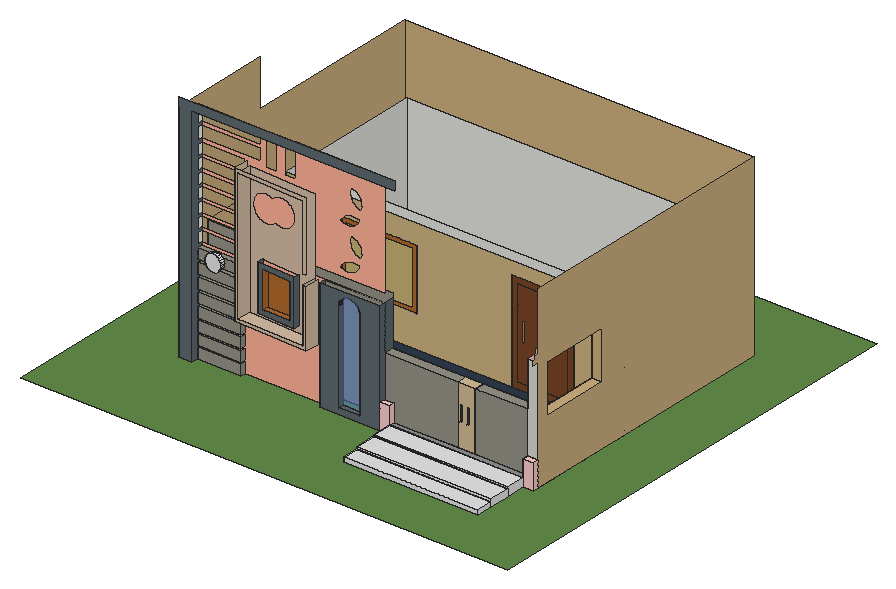
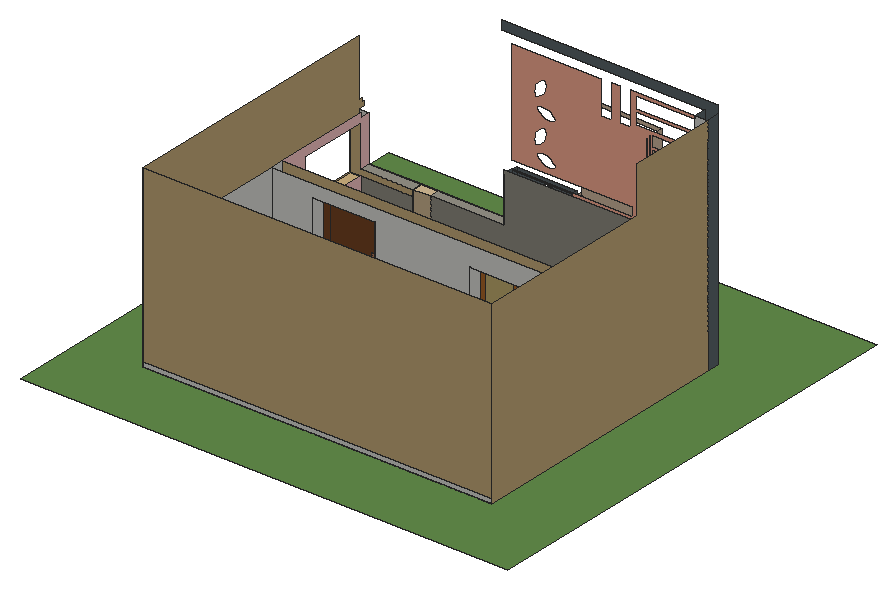
# SketchUp Ruby script. Lengths in inches.
U = 1.inch
M = Sketchup.active_model
def pt(a) = Geom::Point3d.new(a.map { |v| v * U })
def face(e, loops, mat)
  f = e.add_face(loops[0].map { |a| pt(a) })
  loops[1..].each { |l| e.add_face(l.map { |a| pt(a) }).erase! }
  f.material = f.back_material = mat if mat
  f
end
# faces: each face lists its corners as indices into pts; further lists are holes
def faces(e, pts, list, mat = nil) = list.each { |f| face(e, (f[0].is_a?(Array) ? f : [f]).map { |l| l.map { |i| pts[i] } }, mat) }
# xy, xz, yz: faces in a plane at the given z, y or x. An outline is a flat list of corners, or four numbers for a rectangle; further outlines are holes
def ring(l) = l.size == 4 ? [[l[0], l[1]], [l[2], l[1]], [l[2], l[3]], [l[0], l[3]]] : l.each_slice(2).to_a
def flat(e, list, mat, &to3) = list.each { |f| face(e, (f[0].is_a?(Array) ? f : [f]).map { |l| ring(l).map { |u, v| to3.(u, v) } }, mat) }
def xy(e, z, list, mat = nil) = flat(e, list, mat) { |x, y| [x, y, z] }
def xz(e, y, list, mat = nil) = flat(e, list, mat) { |x, z| [x, y, z] }
def yz(e, x, list, mat = nil) = flat(e, list, mat) { |y, z| [x, y, z] }
def lines(e, pts, list) = list.each { |a, b| e.add_line(pt(pts[a]), pt(pts[b])) }
# prism: a flat outline (further loops are holes) pulled along v
def prism(e, loops, v, mat = nil)
  f = face(e, loops, mat); d = Geom::Vector3d.new(v.map { |x| x * U })
  f.pushpull(f.normal.samedirection?(d) ? d.length : -d.length)
end
def box(e, o, s, mat = nil) = prism(e, [[o, [o[0] + s[0], o[1], o[2]], [o[0] + s[0], o[1] + s[1], o[2]], [o[0], o[1] + s[1], o[2]]]], [0, 0, s[2]], mat)
def at(x, y, z, deg = 0) = Geom::Transformation.translation(pt([x, y, z])) * Geom::Transformation.rotation(ORIGIN, Z_AXIS, deg.degrees)
def axes(o, x, y, z) = Geom::Transformation.new([*x, 0, *y, 0, *z, 0, *pt(o).to_a, 1])
def part(name) = M.definitions.add(name)
# library, detail: a bought-in or finely detailed component or shape, given as its bounding box
def library(name, o, s) = part(name).tap { |d| box(d.entities, o, s) }
def detail(e, o, s) = box(e.add_group.entities, o, s)
def put(e, d, t, mat = nil) = e.add_instance(d, t).tap { |i| i.material = mat if mat }
def group(e, t, mat = nil) = e.add_group.tap { |g| g.transformation = t; g.material = mat if mat }.entities
root = M.entities
M.materials.add("[Blacktop Old 02]").color = [143, 145, 145]
M.materials.add("[Color A01]").color = [255, 204, 204]
M.materials.add("[Color B02]").color = [255, 178, 153]
M.materials.add("[Formica Beige]").color = [211, 187, 149]
M.materials.add("[Formica Graystone]").color = [149, 146, 135]
M.materials.add("[Formica Laminate Dark]").color = [50, 53, 60]
M.materials.add("[Formica Laminate Light]").color = [213, 189, 164]
M.materials.add("[Formica Speckled Grey]").color = [94, 105, 111]
M.materials.add("[Leather Blue]").color = [45, 57, 74]
M.materials.add("[Polished Concrete Old]").color = [229, 229, 229]
M.materials.add("[Stone Sandstone Ashlar Light]").color = [206, 178, 128]
M.materials.add("[Terrazzo Tile Light]").color = [219, 217, 210]
M.materials.add("[Translucent Glass Blue]").color = [100, 149, 237]
M.materials["[Translucent Glass Blue]"].alpha = 0.5
M.materials.add("[Vegetation Grass Artificial]").color = [98, 140, 74]
M.materials.add("[Window Covering 02]").color = [199, 178, 115]
M.materials.add("[Wood Bamboo]").color = [177, 105, 43]
M.materials.add("[Wood Floor Light]").color = [204, 176, 127]
M.materials.add("[Wood Veneer 01]").color = [120, 70, 37]
M.materials.add("[Wood Veneer 02]").color = [190, 128, 91]
xy(root,0,[[652.51,124.47,963.43,160.81],[652.51,160.81,963.43,210.65],[652.51,210.65,963.43,256.01],[176.71,240.39,205.21,269.01],[491.29,256.01,491.29,269.01,307.34,269.01,307.34,257.39,205.21,257.39,205.21,269.01,176.71,269.01,176.71,894.96,987.53,894.96,987.53,256.01]])
xy(root,0,[[[0,0,1133.3125,1068.5625],[652.51,124.47,963.43,256.01],[176.71,240.39,205.21,269.01]]],"[Vegetation Grass Artificial]")
xy(root,9,[[963.43,269.01,987.53,293.12],[200.82,520.41,724.72,550.03],[724.72,520.41,868.85,550.03],[868.85,520.41,963.43,550.03],[200.82,550.03,963.43,870.85]])
xy(root,9,[[200.82,293.12,963.43,520.41]],"[Leather Blue]")
xy(root,10.8125,[[652.51,124.47,963.43,160.81]],"[Polished Concrete Old]")
xy(root,13.61,[[533.89,256.01,583.26,269.01]],"[Formica Speckled Grey]")
xy(root,15.875,[[652.51,160.81,963.43,210.65]],"[Polished Concrete Old]")
xy(root,19.25,[[652.51,256.01,963.43,269.01]],"[Blacktop Old 02]")
xy(root,19.25,[[841.49,269.01,963.43,293.12]],"[Color A01]")
xy(root,19.25,[[652.51,210.65,963.43,256.01]],"[Polished Concrete Old]")
xy(root,24,[[205.21,257.39,307.34,269.01]],"[Formica Graystone]")
xy(root,27.52,[[205.21,257.39,307.34,269.01]],"[Formica Graystone]")
xy(root,51.52,[[205.21,257.39,307.34,269.01]],"[Formica Graystone]")
xy(root,56.52,[[205.21,257.39,307.34,269.01]],"[Formica Graystone]")
xy(root,59.0625,[[630.73,256.01,652.51,269.01],[963.43,256.01,987.53,269.01]],"[Color A01]")
xy(root,80.52,[[205.21,257.39,307.34,269.01]],"[Formica Graystone]")
xy(root,83.125,[[330.4375,520.41,503.625,550.03]])
xy(root,85.21,[[205.21,257.39,307.34,269.01]],"[Formica Graystone]")
xy(root,109.21,[[205.21,257.39,307.34,269.01]],"[Formica Graystone]")
xy(root,115.21,[[205.21,257.39,307.34,269.01]],"[Formica Graystone]")
xy(root,124.35,[[479.36,228.58,309.09,236.05,310.54,269.01,480.8,261.55]],"[Formica Laminate Light]")
xy(root,131.76,[[471.96,228.91,473.4,261.88,317.94,268.69,316.5,235.72]],"[Formica Laminate Light]")
xy(root,139.21,[[205.21,257.39,307.34,269.01]],"[Formica Graystone]")
xy(root,140.16,[[963.43,293.12,987.53,454.16]],"[Wood Floor Light]")
xy(root,145.83,[[205.21,257.39,307.34,269.01]],"[Formica Graystone]")
xy(root,146.87,[[436.06,250.0625,348.76,253.89,349.35,267.3125,436.64,263.49]],"[Formica Speckled Grey]")
xy(root,155.65,[[800.41,269.01,841.49,293.12]],"[Formica Beige]")
xy(root,155.65,[[630.73,269.01,800.41,293.12],[841.49,269.01,963.43,293.12]],"[Formica Graystone]")
xy(root,158.32,[[424.62,250.56,425.21,263.99,360.79,266.8125,360.2,253.39]],"[Wood Bamboo]")
xy(root,169.83,[[205.21,257.39,307.34,269.01]],"[Formica Graystone]")
xy(root,176.46,[[205.21,257.39,307.34,269.01]],"[Formica Graystone]")
xy(root,200.46,[[205.21,257.39,307.34,269.01]],"[Formica Graystone]")
xy(root,225.3125,[[330.4375,520.41,503.625,550.03]])
xy(root,231.08,[[205.21,257.39,307.34,269.01]],"[Formica Graystone]")
xz(root,124.47,[[652.51,0,963.43,10.8125]],"[Polished Concrete Old]")
xz(root,160.81,[[652.51,0,963.43,10.8125]])
xz(root,160.81,[[652.51,10.8125,963.43,15.875]],"[Polished Concrete Old]")
xz(root,210.65,[[652.51,0,963.43,15.875]])
xz(root,210.65,[[652.51,15.875,963.43,19.25]],"[Polished Concrete Old]")
xz(root,240.39,[[176.71,0,205.21,0,205.21,522.12,678.16,522.12,678.16,542.5625,176.71,542.5625]],"[Formica Speckled Grey]")
xz(root,246.45,[[249.96,200.625,254.76,201.25,259.24,203.11,263.08,206.05,263.87,207.08,266.02,209.89,267.875,214.37,268.51,219.17,267.875,223.97,266.02,228.4375,263.99,231.08,263.08,232.28,259.24,235.23,254.76,237.08,249.96,237.71,245.16,237.08,240.69,235.23,236.85,232.28,235.94,231.08,233.9,228.4375,232.05,223.97,231.42,219.17,232.05,214.37,233.9,209.89,236.0625,207.08,236.85,206.05,240.69,203.11,245.16,201.25]],"[Polished Concrete Old]")
xz(root,256.01,[[630.73,0,652.51,59.0625],[963.43,0,987.53,59.0625]],"[Color A01]")
xz(root,256.01,[[[491.29,0,630.73,259.36],[533.89,13.61,533.89,224.73,533.92,226.02,534.02,227.3125,534.19,228.59,534.43,229.86,534.73,231.12,535.1,232.36,535.53,233.58,536.02,234.77,536.58,235.9375,537.2,237.07,537.87,238.18,538.6,239.24,539.39,240.27,540.23,241.25,541.12,242.1875,542.06,243.08,543.04,243.92,544.07,244.7,545.13,245.4375,546.23,246.11,547.37,246.73,548.54,247.28,549.73,247.78,550.95,248.21,552.1875,248.58,553.44,248.88,554.72,249.11,556,249.28,557.29,249.38,558.58,249.42,559.87,249.38,561.16,249.28,562.4375,249.11,563.71,248.88,564.97,248.58,566.21,248.21,567.42,247.78,568.62,247.28,569.79,246.73,570.92,246.11,572.02,245.4375,573.09,244.7,574.11,243.92,575.1,243.08,576.03,242.1875,576.92,241.25,577.76,240.27,578.55,239.24,579.28,238.18,579.96,237.07,580.57,235.9375,581.13,234.77,581.625,233.58,582.06,232.36,582.42,231.12,582.73,229.86,582.96,228.59,583.13,227.3125,583.23,226.02,583.26,224.73,583.26,13.61]],[652.51,0,963.43,19.25]],"[Formica Speckled Grey]")
xz(root,257.39,[[235.94,231.08,236.85,232.28,240.69,235.23,245.16,237.08,249.96,237.71,254.76,237.08,259.24,235.23,263.08,232.28,263.99,231.08]])
xz(root,257.39,[[205.21,0,307.34,24],[205.21,27.52,307.34,51.52],[205.21,56.52,307.34,80.52],[205.21,85.21,307.34,109.21],[205.21,115.21,307.34,139.21],
  [205.21,145.83,307.34,169.83],[205.21,176.46,307.34,200.46],[205.21,207.08,236.0625,207.08,233.9,209.89,232.05,214.37,231.42,219.17,232.05,223.97,233.9,228.4375,235.94,231.08,205.21,231.08],[263.87,207.08,307.34,207.08,307.34,231.08,263.99,231.08,266.02,228.4375,267.875,223.97,268.51,219.17,267.875,214.37,266.02,209.89]],"[Formica Graystone]")
xz(root,269.01,[[176.71,0,205.21,522.12],[963.43,9,987.53,59.0625]])
xz(root,269.01,[[[307.34,0,491.29,0,491.29,259.36,630.73,259.36,630.73,261.0625,350.6,261.0625,350.6,280.3125,630.73,280.3125,630.73,522.12,424.625,522.12,424.625,445.43,399.125,445.43,399.125,522.12,380.1875,522.12,380.1875,445.43,354.6875,445.43,354.6875,522.12,205.21,522.12,205.21,515.1,342.46,515.1,342.46,488.66,205.21,488.66,205.21,481.6,342.46,481.6,342.46,455.16,205.21,455.16,205.21,445.46,307.34,445.46,307.34,421.46,205.21,421.46,205.21,414.83,307.34,414.83,307.34,390.83,205.21,390.83,205.21,384.21,307.34,384.21,307.34,360.21,205.21,360.21,205.21,353.58,307.34,353.58,307.34,329.58,205.21,329.58,205.21,322.96,307.34,322.96,307.34,298.96,205.21,298.96,205.21,292.33,307.34,292.33,307.34,268.33,205.21,268.33,205.21,261.71,307.34,261.71,307.34,237.71,205.21,237.71,205.21,231.08,307.34,231.08,307.34,207.08,205.21,207.08,205.21,200.46,307.34,200.46,307.34,176.46,205.21,176.46,205.21,169.83,307.34,169.83,307.34,145.83,205.21,145.83,205.21,139.21,307.34,139.21,307.34,115.21,205.21,115.21,205.21,109.21,307.34,109.21,307.34,85.21,205.21,85.21,205.21,80.52,307.34,80.52,307.34,56.52,205.21,56.52,205.21,51.52,307.34,51.52,307.34,27.52,205.21,27.52,205.21,24,307.34,24],[545.83,390.61,541.09,390.87,536.44,391.87,532.01,393.57,527.89,395.95,530.06,399.98,532.74,403.67,535.9,406.98,539.47,409.82,543.39,412.17,547.59,413.96,551.99,415.17,556.52,415.78,561.09,415.78,565.61,415.16,570.02,413.94,574.21,412.13,572.47,407.71,570.07,403.61,567.05,399.94,563.5,396.78,559.51,394.21,555.16,392.3,550.5625,391.09],[545.83,293.67,541.09,293.93,536.44,294.93,532.01,296.64,527.89,299.02,530.06,303.04,532.74,306.74,535.9,310.04,539.47,312.89,543.39,315.23,547.59,317.02,551.99,318.23,556.52,318.84,561.09,318.84,565.61,318.22,570.02,317,574.21,315.2,572.47,310.77,570.07,306.68,567.05,303,563.5,299.84,559.51,297.28,555.16,295.36,550.5625,294.15],[577.86,330.87,573.2,331.8,568.74,333.44,564.59,335.76,560.86,338.69,557.62,342.17,554.97,346.12,552.96,350.42,551.65,354.99,551.07,359.71,551.23,364.46,552.125,369.125,553.74,373.59,558.08,372.18,562.19,370.19,566,367.67,569.4375,364.66,572.4375,361.21,574.95,357.4,576.92,353.28,578.32,348.93,579.125,344.43,579.32,339.87,578.89,335.32],[577.86,431.06,573.2,431.99,568.74,433.63,564.59,435.95,560.86,438.88,557.62,442.36,554.97,446.3,552.96,450.61,551.65,455.18,551.07,459.89,551.23,464.64,552.125,469.3125,553.74,473.78,558.08,472.37,562.19,470.38,566,467.86,569.4375,464.85,572.4375,461.4,574.95,457.59,576.92,453.47,578.32,449.12,579.125,444.62,579.32,440.06,578.89,435.51]]],"[Color B02]")
xz(root,269.01,[[[800.41,19.25,841.49,155.65],[805.56,73.97,811.87,111.16],[821.68,73.97,827.99,111.16]]],"[Formica Beige]")
xz(root,269.01,[[652.51,19.25,800.41,19.25,800.41,155.65,630.73,155.65,630.73,59.0625,652.51,59.0625],[841.49,19.25,963.43,155.65]],"[Formica Graystone]")
xz(root,269.01,[[805.56,73.97,811.87,111.16],[821.68,73.97,827.99,111.16]],"[Formica Laminate Dark]")
xz(root,269.01,[[963.43,59.0625,987.53,261.0625]],"[Terrazzo Tile Light]")
xz(root,269.01,[[533.89,13.61,583.26,13.61,583.26,224.73,583.23,226.02,583.13,227.3125,582.96,228.59,582.73,229.86,582.42,231.12,582.06,232.36,581.625,233.58,581.13,234.77,580.57,235.9375,579.96,237.07,579.28,238.18,578.55,239.24,577.76,240.27,576.92,241.25,576.03,242.1875,575.1,243.08,574.11,243.92,573.09,244.7,572.02,245.4375,570.92,246.11,569.79,246.73,568.62,247.28,567.42,247.78,566.21,248.21,564.97,248.58,563.71,248.88,562.4375,249.11,561.16,249.28,559.87,249.38,558.58,249.42,557.29,249.38,556,249.28,554.72,249.11,553.44,248.88,552.1875,248.58,550.95,248.21,549.73,247.78,548.54,247.28,547.37,246.73,546.23,246.11,545.13,245.4375,544.07,244.7,543.04,243.92,542.06,243.08,541.12,242.1875,540.23,241.25,539.39,240.27,538.6,239.24,537.87,238.18,537.2,237.07,536.58,235.9375,536.02,234.77,535.53,233.58,535.1,232.36,534.73,231.12,534.43,229.86,534.19,228.59,534.02,227.3125,533.92,226.02,533.89,224.73]],"[Translucent Glass Blue]")
xz(root,293.12,[[963.43,9,987.53,140.16]])
xz(root,293.12,[[630.73,9,630.73,19.25,800.41,19.25,800.41,155.65,841.49,155.65,841.49,19.25,963.43,19.25,963.43,9]],"[Formica Beige]")
xz(root,293.12,[[200.82,9,200.82,271.3125,630.73,271.3125,630.73,155.65,800.41,155.65,800.41,19.25,630.73,19.25,630.73,9],[841.49,19.25,963.43,140.16]],"[Formica Graystone]")
xz(root,293.12,[[841.49,140.16,841.49,155.65,963.43,155.65,963.43,251.7,987.53,251.7,987.53,140.16]],"[Wood Floor Light]")
xz(root,454.16,[[963.43,140.16,987.53,251.7]],"[Wood Floor Light]")
xz(root,520.41,[[[200.82,9,724.72,9,724.72,242.2,868.85,242.2,868.85,9,963.43,9,963.43,271.3125,200.82,271.3125],[330.4375,83.125,503.625,225.3125]]],"[Stone Sandstone Ashlar Light]")
xz(root,520.41,[[340.5625,93.25,409.01,215.1875],[425.5,93.25,493.5,215.1875]],"[Window Covering 02]")
xz(root,520.41,[[[330.4375,83.125,503.625,225.3125],[340.5625,93.25,493.5,215.1875]],[409.01,93.25,425.5,215.1875]],"[Wood Bamboo]")
xz(root,520.41,[[[724.72,9,868.85,242.2],[739.6875,23.96,853.88,227.23]],[[739.6875,23.96,853.88,227.23],[747.59,107.64,755.03,154.64]]],"[Wood Veneer 01]")
xz(root,520.41,[[747.59,107.64,755.03,154.64]],"[Wood Veneer 02]")
xz(root,550.03,[[[200.82,9,200.82,271.3125,963.43,271.3125,963.43,9,868.85,9,868.85,242.2,724.72,242.2,724.72,9],[330.4375,83.125,503.625,225.3125]]])
xz(root,870.85,[[200.82,9,963.43,271.3125]])
xz(root,894.96,[[176.71,0,987.53,9]])
xz(root,894.96,[[176.71,9,987.53,414.1875]],"[Wood Floor Light]")
yz(root,176.71,[[240.39,0,269.01,522.12]],"[Formica Speckled Grey]")
yz(root,176.71,[[269.01,0,269.01,522.12,475.31,522.12,475.31,414.1875,894.96,414.1875,894.96,0]],"[Wood Floor Light]")
yz(root,200.82,[[520.41,9,550.03,271.3125],[550.03,9,870.85,271.3125]])
yz(root,200.82,[[293.12,9,520.41,271.3125]],"[Stone Sandstone Ashlar Light]")
yz(root,205.21,[[257.39,0,269.01,24],[257.39,27.52,269.01,51.52],[257.39,56.52,269.01,80.52],[257.39,85.21,269.01,109.21],[257.39,115.21,269.01,139.21],
  [257.39,145.83,269.01,169.83],[257.39,176.46,269.01,200.46],[257.39,207.08,269.01,231.08]])
yz(root,205.21,[[240.39,0,257.39,0,257.39,24,269.01,24,269.01,27.52,257.39,27.52,257.39,51.52,269.01,51.52,269.01,56.52,257.39,56.52,257.39,80.52,269.01,80.52,269.01,85.21,257.39,85.21,257.39,109.21,269.01,109.21,269.01,115.21,257.39,115.21,257.39,139.21,269.01,139.21,269.01,145.83,257.39,145.83,257.39,169.83,269.01,169.83,269.01,176.46,257.39,176.46,257.39,200.46,269.01,200.46,269.01,207.08,257.39,207.08,257.39,231.08,269.01,231.08,269.01,237.71,257.39,237.71,257.39,261.71,269.01,261.71,269.01,268.33,257.39,268.33,257.39,292.33,269.01,292.33,269.01,298.96,257.39,298.96,257.39,322.96,269.01,322.96,269.01,329.58,257.39,329.58,257.39,353.58,269.01,353.58,269.01,360.21,257.39,360.21,257.39,384.21,269.01,384.21,269.01,390.83,257.39,390.83,257.39,414.83,269.01,414.83,269.01,421.46,257.39,421.46,257.39,445.46,269.01,445.46,269.01,455.16,257.39,455.16,257.39,481.6,269.01,481.6,269.01,488.66,257.39,488.66,257.39,515.1,269.01,515.1,269.01,522.12,240.39,522.12]],"[Formica Speckled Grey]")
yz(root,307.34,[[257.39,145.83,269.01,169.83],[257.39,176.46,269.01,200.46],[257.39,207.08,269.01,231.08]])
yz(root,307.34,[[257.39,0,269.01,24],[257.39,27.52,269.01,51.52],[257.39,56.52,269.01,80.52],[257.39,85.21,269.01,109.21],[257.39,115.21,269.01,139.21]],"[Formica Graystone]")
yz(root,330.4375,[[520.41,83.125,550.03,225.3125]])
yz(root,491.29,[[256.01,0,269.01,259.36]],"[Formica Speckled Grey]")
yz(root,503.625,[[520.41,83.125,550.03,225.3125]])
yz(root,533.89,[[256.01,13.61,269.01,224.73]],"[Formica Speckled Grey]")
yz(root,583.26,[[256.01,13.61,269.01,224.73]],"[Formica Speckled Grey]")
yz(root,630.73,[[256.01,59.0625,269.01,259.36],[269.01,155.65,293.12,261.0625]],"[Formica Speckled Grey]")
yz(root,652.51,[[256.01,19.25,269.01,59.0625]],"[Color A01]")
yz(root,652.51,[[124.47,0,160.81,10.8125],[160.81,0,210.65,15.875],[210.65,0,256.01,19.25]],"[Polished Concrete Old]")
yz(root,724.72,[[520.41,9,550.03,242.2]])
yz(root,841.49,[[269.01,19.25,293.12,155.65]],"[Color A01]")
yz(root,868.85,[[520.41,9,550.03,242.2]])
yz(root,963.43,[[269.01,9,293.12,19.25],[520.41,9,550.03,271.3125],[550.03,9,870.85,271.3125]])
yz(root,963.43,[[293.12,9,293.12,140.16,454.16,140.16,454.16,251.7,293.12,251.7,293.12,155.65,269.01,155.65,269.01,261.0625,293.12,261.0625,293.12,271.3125,520.41,271.3125,520.41,9],[256.01,19.25,269.01,59.0625]],"[Color A01]")
yz(root,963.43,[[124.47,0,160.81,10.8125],[160.81,0,210.65,15.875],[210.65,0,256.01,19.25]],"[Polished Concrete Old]")
yz(root,987.53,[[256.01,0,269.01,59.0625]],"[Color A01]")
yz(root,987.53,[[[269.01,0,894.96,0,894.96,414.1875,269.01,414.1875,269.01,280.3125,258.7,280.3125,258.7,271.3125,252.2,271.3125,252.2,261.0625,269.01,261.0625],[293.12,140.16,454.16,251.7]]],"[Wood Floor Light]")
p = [[479.36,228.58,124.35],[479.36,228.58,258.72],[471.96,228.91,258.72],[471.96,228.91,131.76],[316.5,235.72,131.76],[316.5,235.72,435.11],
  [471.96,228.91,435.11],[471.96,228.91,283.43],[479.36,228.58,283.43],[479.36,228.58,442.52],[309.09,236.05,442.52],[309.09,236.05,124.35],
  [480.8,261.55,124.35],[480.8,261.55,258.72],[310.54,269.01,442.52],[310.54,269.01,124.35],[473.4,261.88,258.72],[473.4,261.88,131.76],
  [317.94,268.69,131.76],[317.94,268.69,435.11],[473.4,261.88,435.11],[473.4,261.88,283.43],[436.64,263.49,253.37],[436.64,263.49,146.87],
  [349.35,267.3125,146.87],[349.35,267.3125,253.37],[372.63,266.29,389.13],[373.35,266.26,388.7],[373.44,266.26,388.8],[375.94,266.15,390.97],
  [378.66,266.03,392.86],[381.55,265.9,394.46],[384.6,265.77,395.75],[387.76,265.63,396.71],[391.01,265.49,397.34],[394.3,265.34,397.62],
  [397.61,265.2,397.56],[400.89,265.06,397.15],[404.11,264.91,396.4],[407.24,264.78,395.32],[410.23,264.65,393.92],[413.06,264.52,392.21],
  [415.7,264.41,390.21],[418.12,264.3,387.95],[420.28,264.21,385.45],[422.18,264.12,382.73],[423.78,264.05,379.83],[425.0625,264,376.79],
  [426.02,263.95,373.62],[426.65,263.93,370.37],[426.93,263.91,367.07],[426.87,263.92,363.76],[426.46,263.93,360.48],[425.71,263.97,357.25],
  [424.63,264.01,354.12],[423.23,264.08,351.125],[421.52,264.15,348.29],[419.53,264.24,345.65],[417.27,264.34,343.23],[414.77,264.45,341.0625],
  [412.06,264.57,339.17],[409.16,264.69,337.57],[406.12,264.83,336.28],[402.95,264.96,335.32],[399.7,265.11,334.69],[396.41,265.25,334.41],
  [393.1,265.4,334.47],[389.82,265.54,334.88],[386.6,265.68,335.63],[383.48,265.82,336.71],[380.48,265.95,338.12],[379.77,265.98,338.55],
  [379.67,265.99,338.44],[377.17,266.09,336.28],[374.46,266.21,334.38],[371.5625,266.34,332.78],[368.52,266.47,331.49],[365.35,266.61,330.53],
  [362.11,266.75,329.9],[358.8125,266.9,329.62],[355.51,267.04,329.68],[352.22,267.1875,330.09],[349,267.33,330.84],[345.88,267.47,331.92],
  [342.88,267.6,333.33],[340.05,267.72,335.04],[337.41,267.84,337.03],[335,267.94,339.3],[332.83,268.04,341.8],[330.9375,268.12,344.51],
  [329.34,268.19,347.41],[328.05,268.25,350.46],[327.09,268.29,353.625],[326.46,268.32,356.875],[326.18,268.33,360.17],[326.24,268.33,363.48],
  [326.65,268.31,366.77],[327.4,268.28,369.99],[328.48,268.23,373.12],[329.89,268.17,376.12],[331.59,268.09,378.95],[333.59,268,381.59],
  [335.85,267.91,384.01],[338.35,267.8,386.18],[341.06,267.68,388.07],[343.95,267.55,389.67],[347,267.42,390.96],[350.16,267.28,391.93],
  [353.41,267.14,392.55],[356.7,266.99,392.84],[360.01,266.85,392.77],[363.29,266.7,392.36],[366.51,266.5625,391.61],[369.64,266.42,390.53],
  [436.06,250.0625,146.87],[436.06,250.0625,253.37],[348.76,253.89,253.37],[348.76,253.89,146.87],[360.2,253.39,158.32],[360.2,253.39,241.92],
  [424.62,250.56,241.92],[424.62,250.56,158.32],[425.21,263.99,241.92],[425.21,263.99,158.32],[360.79,266.8125,158.32],[360.79,266.8125,241.92],
  [245.16,257.39,201.25],[249.96,257.39,200.625],[249.96,246.45,200.625],[245.16,246.45,201.25],[254.76,257.39,201.25],[254.76,246.45,201.25],
  [240.69,257.39,203.11],[240.69,246.45,203.11],[259.24,257.39,203.11],[259.24,246.45,203.11],[236.85,257.39,206.05],[236.85,246.45,206.05],
  [263.08,257.39,206.05],[263.08,246.45,206.05],[236.0625,257.39,207.08],[236.0625,246.45,207.08],[263.87,257.39,207.08],[263.87,246.45,207.08],
  [233.9,257.39,209.89],[233.9,246.45,209.89],[266.02,257.39,209.89],[266.02,246.45,209.89],[232.05,257.39,214.37],[232.05,246.45,214.37],
  [267.875,257.39,214.37],[267.875,246.45,214.37],[231.42,257.39,219.17],[231.42,246.45,219.17],[268.51,257.39,219.17],[268.51,246.45,219.17],
  [232.05,257.39,223.97],[232.05,246.45,223.97],[267.875,257.39,223.97],[267.875,246.45,223.97],[233.9,257.39,228.4375],[233.9,246.45,228.4375],
  [266.02,257.39,228.4375],[266.02,246.45,228.4375],[533.89,269.01,224.73],[533.92,269.01,226.02],[533.92,256.01,226.02],[533.89,256.01,224.73],
  [583.23,269.01,226.02],[583.26,269.01,224.73],[583.26,256.01,224.73],[583.23,256.01,226.02],[534.02,269.01,227.3125],[534.02,256.01,227.3125],
  [583.13,269.01,227.3125],[583.13,256.01,227.3125],[534.19,269.01,228.59],[534.19,256.01,228.59],[582.96,269.01,228.59],[582.96,256.01,228.59],
  [236.85,257.39,232.28],[235.94,257.39,231.08],[235.94,246.45,231.08],[236.85,246.45,232.28],[263.99,257.39,231.08],[263.08,257.39,232.28],
  [263.08,246.45,232.28],[263.99,246.45,231.08],[534.43,269.01,229.86],[534.43,256.01,229.86],[582.73,269.01,229.86],[582.73,256.01,229.86],
  [534.73,269.01,231.12],[534.73,256.01,231.12],[582.42,269.01,231.12],[582.42,256.01,231.12],[535.1,269.01,232.36],[535.1,256.01,232.36],
  [582.06,269.01,232.36],[582.06,256.01,232.36],[240.69,257.39,235.23],[240.69,246.45,235.23],[259.24,257.39,235.23],[259.24,246.45,235.23],
  [535.53,269.01,233.58],[535.53,256.01,233.58],[581.625,269.01,233.58],[581.625,256.01,233.58],[536.02,269.01,234.77],[536.02,256.01,234.77],
  [581.13,269.01,234.77],[581.13,256.01,234.77],[536.58,269.01,235.9375],[536.58,256.01,235.9375],[580.57,269.01,235.9375],[580.57,256.01,235.9375],
  [245.16,257.39,237.08],[245.16,246.45,237.08],[254.76,257.39,237.08],[254.76,246.45,237.08],[537.2,269.01,237.07],[537.2,256.01,237.07],
  [579.96,269.01,237.07],[579.96,256.01,237.07],[249.96,257.39,237.71],[249.96,246.45,237.71],[537.87,269.01,238.18],[537.87,256.01,238.18],
  [579.28,269.01,238.18],[579.28,256.01,238.18],[963.43,520.41,9],[987.53,520.41,9],[963.43,520.41,140.16],[987.53,520.41,140.16]]
faces(root,p,[[0,1,2,3,4,5,6,7,8,9,10,11],[12,13,1,0],[14,15,11,10],[16,17,3,2],[18,19,5,4],[[20,19,18,17,16,21],[22,23,24,25],[26,27,28,29,30,31,32,33,34,35,36,37,38,39,40,41,42,43,44,45,46,47,48,49,50,51,52,53,54,55,56,57,58,59,60,61,62,63,64,65,66,67,68,69,70,71,72,73,74,75,76,77,78,79,80,81,82,83,84,85,86,87,88,89,90,91,92,93,94,95,96,97,98,99,100,101,102,103,104,105,106,107,108,109,110,111,112,113]]],"[Formica Laminate Light]")
faces(root,p,[[[114,115,116,117],[118,119,120,121]],[23,22,115,114],[25,24,117,116],[164,165,166,167],[168,169,170,171],[165,172,173,166],[174,168,171,175],[172,176,177,173],
  [178,174,175,179],[176,188,189,177],[190,178,179,191],[188,192,193,189],[194,190,191,195],[192,196,197,193],[198,194,195,199],[196,204,205,197],
  [206,198,199,207],[204,208,209,205],[210,206,207,211],[208,212,213,209],[214,210,211,215],[212,220,221,213],[222,214,215,223],[220,226,227,221],
  [228,222,223,229]],"[Formica Speckled Grey]")
faces(root,p,[[122,123,121,120],[124,125,119,118],[125,124,123,122]],"[Wood Bamboo]")
faces(root,p,[[126,127,128,129],[127,130,131,128],[132,126,129,133],[130,134,135,131],[136,132,133,137],[134,138,139,135],[140,136,137,141],[138,142,143,139],
  [144,140,141,145],[142,146,147,143],[148,144,145,149],[146,150,151,147],[152,148,149,153],[150,154,155,151],[156,152,153,157],[154,158,159,155],
  [160,156,157,161],[158,162,163,159],[180,181,160,161,182,183],[162,184,185,186,187,163],[200,180,183,201],[185,202,203,186],[216,200,201,217],[202,218,219,203],
  [224,216,217,225],[218,224,225,219]],"[Polished Concrete Old]")
lines(root,p,[[230,231],[232,233]])
